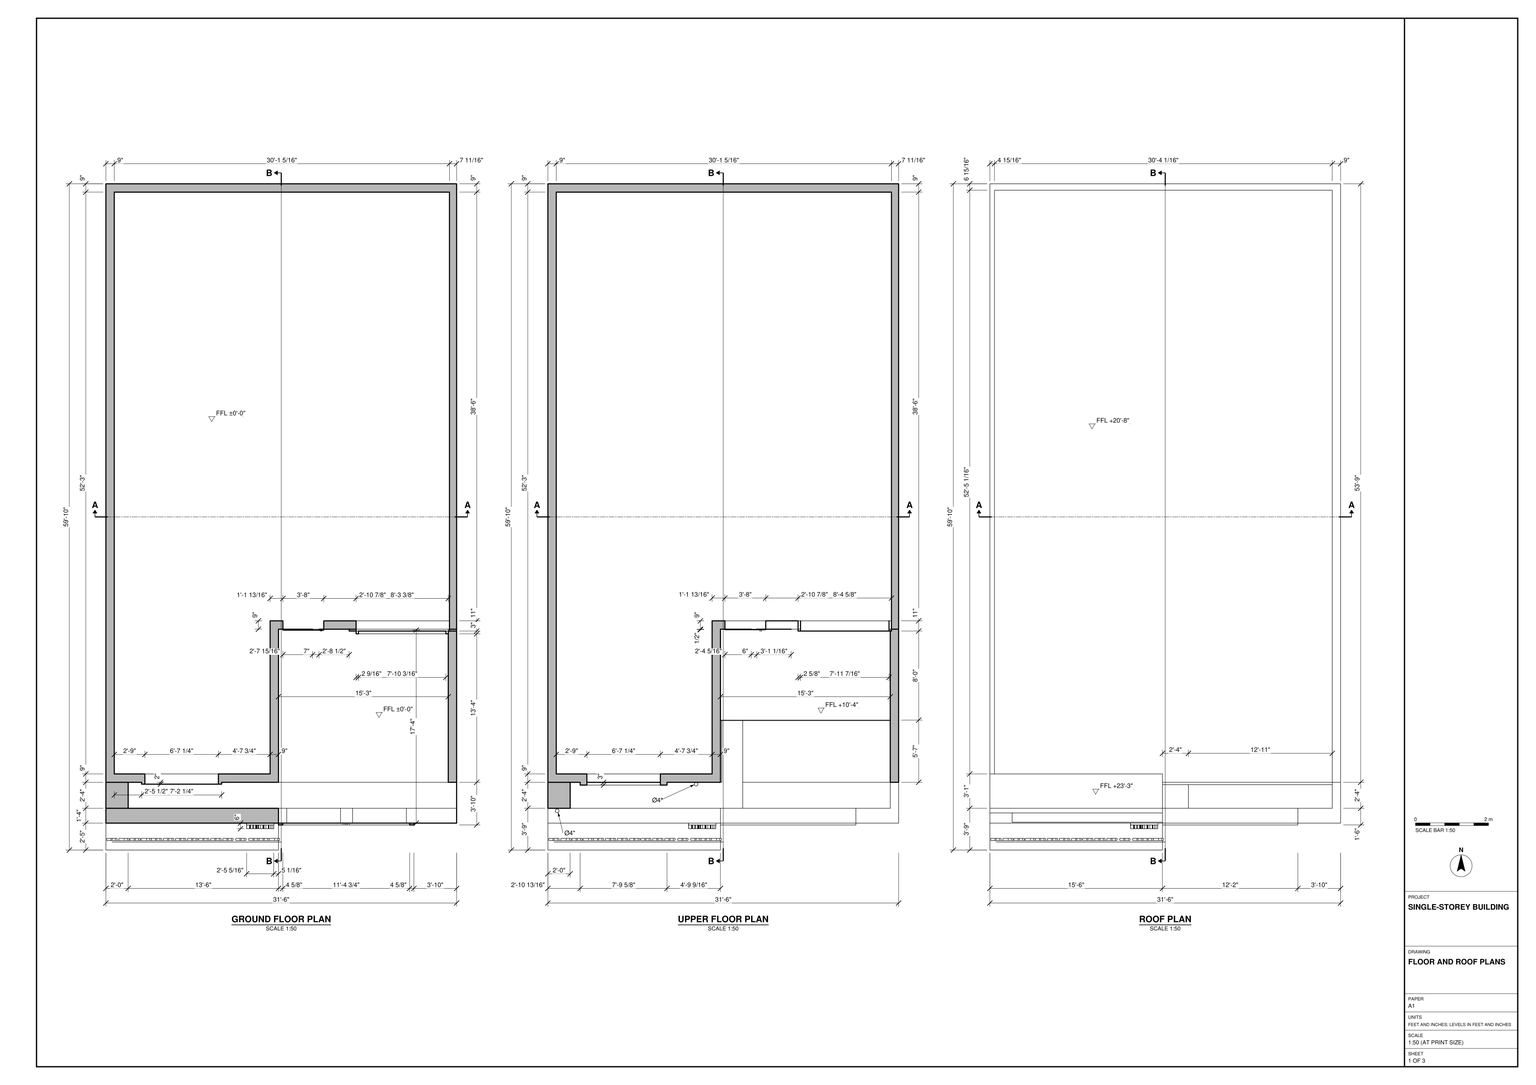
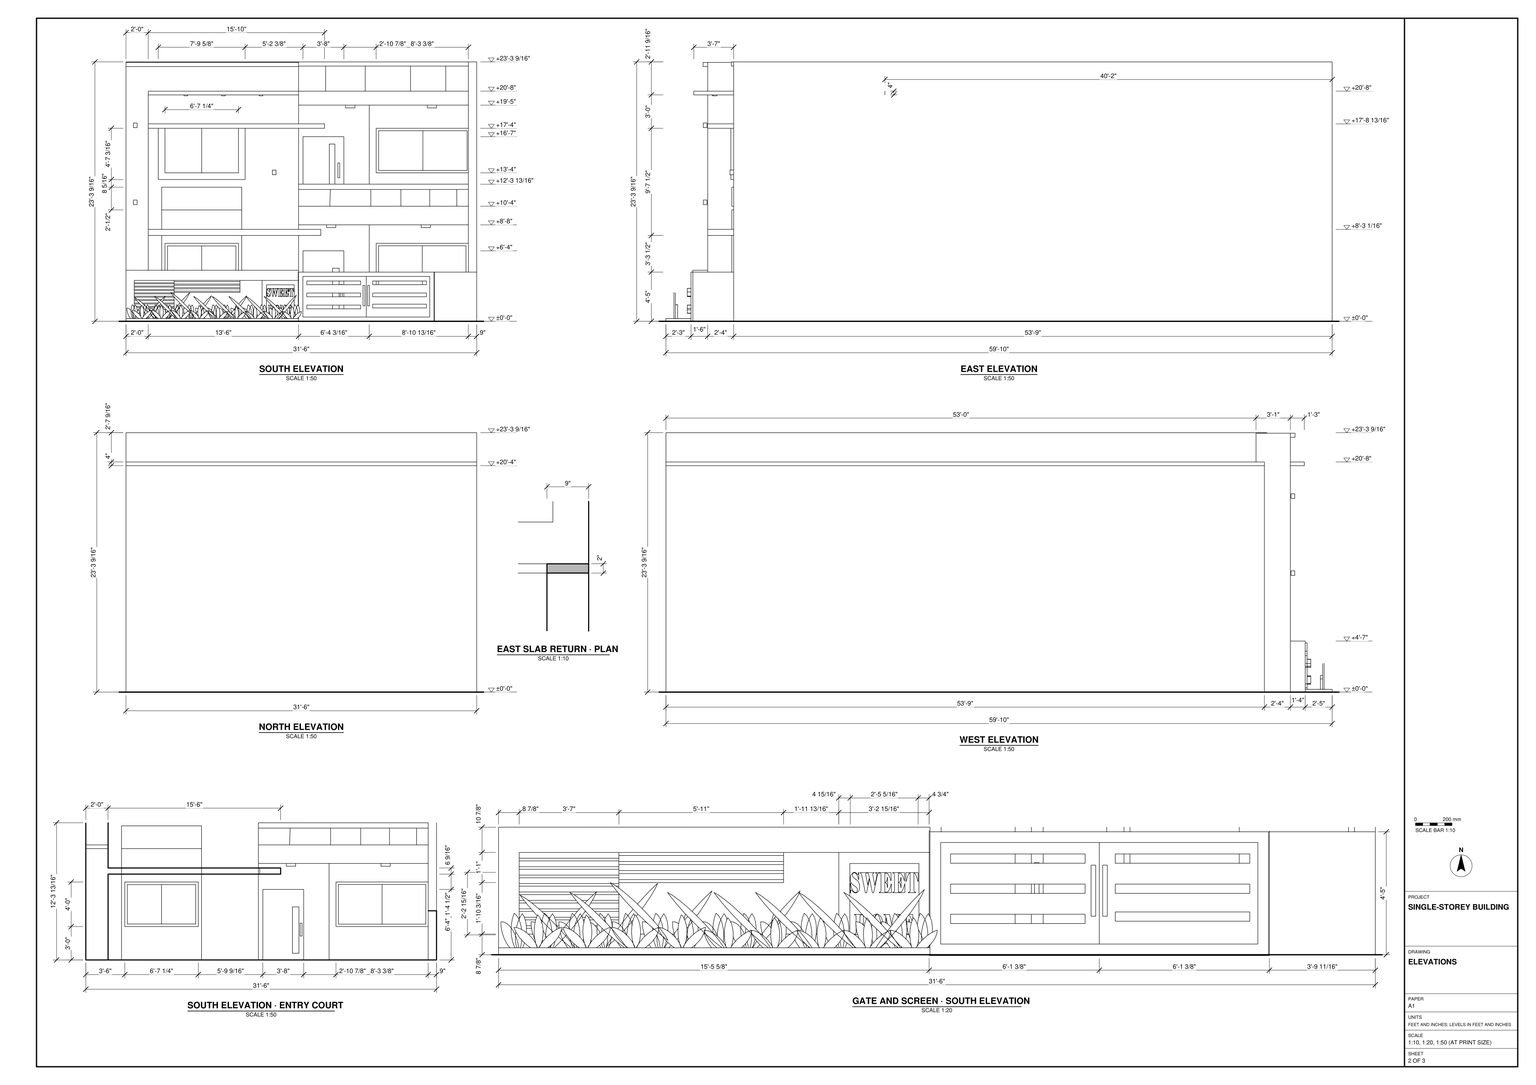
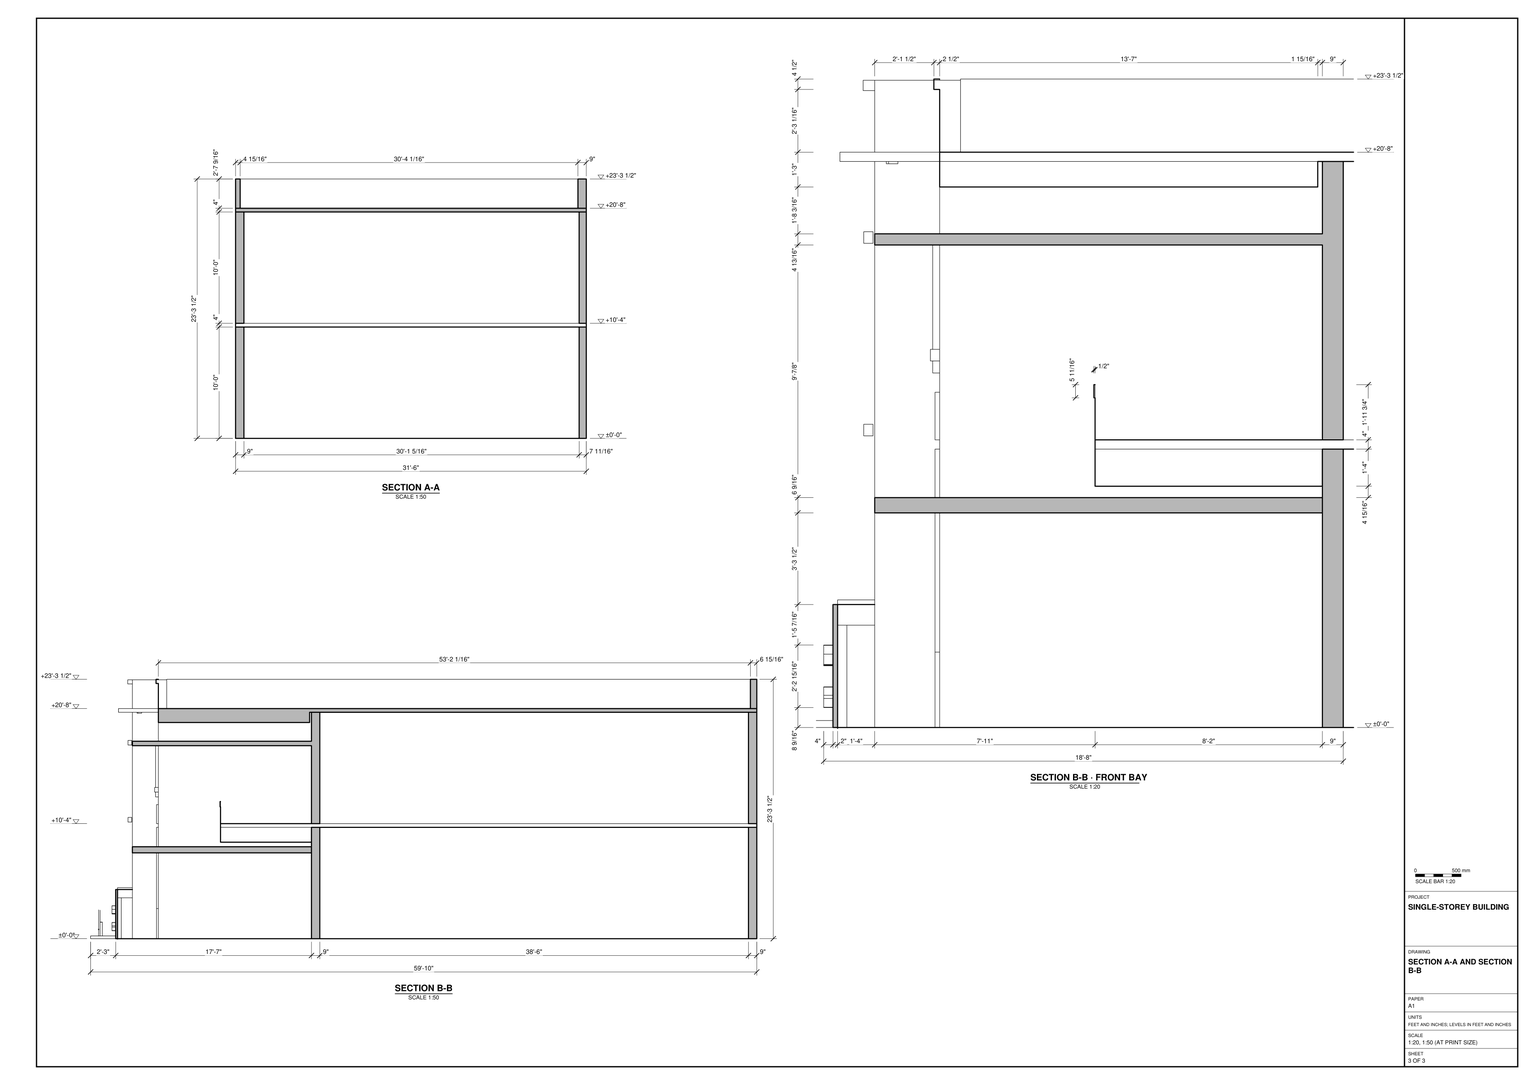
Build the house and its south entry court in SketchUp from task_files/diagram_01.pdf. Work in feet and inches. The overall model is 31'-6" across the frontage, 59'-10" from front to back and 23'-3 7/8" high. Set the ground floor at ±0'-0", the upper floor at +10'-4" and the main roof surface at +20'-8".

Use the floor plans to lay out the long side walls, the rear wall and the stepped south frontage. Follow the wall thicknesses as drawn. The west bay extends toward the street, while the door and wide window to its east sit farther back in the court. Use the sections to distinguish the upper floor slab and its projection into the court from the thinner shading ledges. Model the flat roof and its raised parapet. Use the south elevations to place the framed windows, doors and projecting bands at both storeys.

At the street edge, model the screen and its planting strip on the left and the paired gate leaves on the right, as seen from the south. Decor and loose items, including the plants, may be any suitable library components. Keep walls, slabs, roof elements and individual fitted pieces in separate groups or components, and use components for repeated parts. Save one SketchUp model as output_files/two_storey_house_with_a_screened_entry_court.skp.

# SketchUp Ruby script. Lengths in inches.
U = 1.inch
M = Sketchup.active_model
def pt(a) = Geom::Point3d.new(a.map { |v| v * U })
def face(e, loops, mat)
  f = e.add_face(loops[0].map { |a| pt(a) })
  loops[1..].each { |l| e.add_face(l.map { |a| pt(a) }).erase! }
  f.material = f.back_material = mat if mat
  f
end
# faces: each face lists its corners as indices into pts; further lists are holes
def faces(e, pts, list, mat = nil) = list.each { |f| face(e, (f[0].is_a?(Array) ? f : [f]).map { |l| l.map { |i| pts[i] } }, mat) }
# xy, xz, yz: faces in a plane at the given z, y or x. An outline is a flat list of corners, or four numbers for a rectangle; further outlines are holes
def ring(l) = l.size == 4 ? [[l[0], l[1]], [l[2], l[1]], [l[2], l[3]], [l[0], l[3]]] : l.each_slice(2).to_a
def flat(e, list, mat, &to3) = list.each { |f| face(e, (f[0].is_a?(Array) ? f : [f]).map { |l| ring(l).map { |u, v| to3.(u, v) } }, mat) }
def xy(e, z, list, mat = nil) = flat(e, list, mat) { |x, y| [x, y, z] }
def xz(e, y, list, mat = nil) = flat(e, list, mat) { |x, z| [x, y, z] }
def yz(e, x, list, mat = nil) = flat(e, list, mat) { |y, z| [x, y, z] }
def lines(e, pts, list) = list.each { |a, b| e.add_line(pt(pts[a]), pt(pts[b])) }
# prism: a flat outline (further loops are holes) pulled along v
def prism(e, loops, v, mat = nil)
  f = face(e, loops, mat); d = Geom::Vector3d.new(v.map { |x| x * U })
  f.pushpull(f.normal.samedirection?(d) ? d.length : -d.length)
end
def box(e, o, s, mat = nil) = prism(e, [[o, [o[0] + s[0], o[1], o[2]], [o[0] + s[0], o[1] + s[1], o[2]], [o[0], o[1] + s[1], o[2]]]], [0, 0, s[2]], mat)
def at(x, y, z, deg = 0) = Geom::Transformation.translation(pt([x, y, z])) * Geom::Transformation.rotation(ORIGIN, Z_AXIS, deg.degrees)
def axes(o, x, y, z) = Geom::Transformation.new([*x, 0, *y, 0, *z, 0, *pt(o).to_a, 1])
def part(name) = M.definitions.add(name)
# library, detail: a bought-in or finely detailed component or shape, given as its bounding box
def library(name, o, s) = part(name).tap { |d| box(d.entities, o, s) }
def detail(e, o, s) = box(e.add_group.entities, o, s)
def put(e, d, t, mat = nil) = e.add_instance(d, t).tap { |i| i.material = mat if mat }
def group(e, t, mat = nil) = e.add_group.tap { |g| g.transformation = t; g.material = mat if mat }.entities
root = M.entities
M.materials.add("Lily_Dark").color = [68, 42, 38]
M.materials.add("[Cladding Siding Tan]").color = [162, 126, 95]
M.materials.add("[Cladding Siding White]").color = [207, 207, 207]
M.materials.add("[Color A02]").color = [255, 153, 153]
M.materials.add("[Color C01]").color = [255, 229, 204]
M.materials.add("[Color D03]").color = [255, 216, 101]
M.materials.add("[Color M00]").color = [255, 255, 255]
M.materials.add("[Color M09]").color = [0, 0, 0]
M.materials.add("[Formica Speckled Grey]").color = [94, 105, 111]
M.materials.add("[Grass Dark Green]").color = [106, 157, 55]
M.materials.add("[Quartz Light Brown]").color = [199, 184, 152]
M.materials.add("[Translucent Glass Gray]").color = [128, 128, 128]
M.materials["[Translucent Glass Gray]"].alpha = 0.5
M.materials.add("[Vegetation Blur 03]").color = [83, 114, 18]
M.materials.add("[Vegetation Grass Artificial]").color = [98, 140, 74]
M.materials.add("[Vegetation Grass]").color = [144, 160, 91]
M.materials.add("[Wood Cherry Original]").color = [152, 86, 42]
M.materials.add("[Wood Lumber ButtJoined]").color = [164, 152, 112]
M.materials.add("[Wood Veneer 01]").color = [120, 70, 37]
M.materials.add("[Wood Veneer 02]").color = [190, 128, 91]
c1 = part("Horizontal screen slat")
box(c1.entities,[0,0,0],[42.97,1,2.5])
c2 = part("Slatted screen panel")
put(c2.entities,c1,at(0,-1,0),"[Wood Cherry Original]")
put(c2.entities,c1,at(0,-1,-3.63),"[Wood Cherry Original]")
put(c2.entities,c1,at(0,-1,-7.27),"[Wood Cherry Original]")
put(c2.entities,c1,at(0,-1,-10.9),"[Wood Cherry Original]")
put(c2.entities,c1,at(0,-1,-14.53),"[Wood Cherry Original]")
put(c2.entities,c1,at(0,-1,-18.17),"[Wood Cherry Original]")
put(c2.entities,c1,at(0,-1,-21.8),"[Wood Cherry Original]")
put(c2.entities,c1,at(0,-1,-25.43),"[Wood Cherry Original]")
put(c2.entities,c1,at(0,-1,-29.07),"[Wood Cherry Original]")
put(c2.entities,c1,at(0,-1,-32.7),"[Wood Cherry Original]")
c3 = library("SWEET  HOME",[-3.58,-8.11,0],[25.68,26.97,6])
c4 = part("Difference\#1")
xy(c4.entities,0,[[38.49,-2,38.49,0,0,0,0,645,378,645,378,165,234.81,165,234.81,174,370.29,174,370.29,636,9,636,9,9,177,9,177,174,190.8,174,190.8,165,186,165,186,0,124.73,0,124.73,-2]],"[Cladding Siding White]")
xy(c4.entities,20.51,[[38.49,-2,124.73,0]],"[Cladding Siding Tan]")
xy(c4.entities,28.81,[[34.8,-3,128.41,0]],"[Cladding Siding White]")
xy(c4.entities,36,[[42,-3,121.22,0],[42,0,121.22,9],[269.66,165,370.29,174]],"[Cladding Siding White]")
xy(c4.entities,75,[[190.8,165,234.81,174]],"[Cladding Siding White]")
xy(c4.entities,84,[[34.8,-3,42,0],[121.22,-3,128.41,0],[42,0,121.22,9],[269.66,165,370.29,174]],"[Cladding Siding White]")
xy(c4.entities,84,[[24,-28,24,0,34.8,0,34.8,-3,42,-3,42,0,121.22,0,121.22,-3,128.41,-3,128.41,0,186,0,186,165,214,165,214,-28]],"[Color M00]")
xy(c4.entities,88.8125,[[24,-28,214,-28,214,165,186,165,186,0,24,0]],"[Color M00]")
xy(c4.entities,120,[[[0,0,186,0,186,165,378,165,378,645,0,645],[9,9,9,636,370.29,636,370.29,174,177,174,177,9]]],"[Cladding Siding White]")
xz(c4.entities,-28,[[24,84,214,88.8125]],"[Color M00]")
xz(c4.entities,-3,[[34.8,28.81,128.41,28.81,128.41,84,121.22,84,121.22,36,42,36,42,84,34.8,84]],"[Formica Speckled Grey]")
xz(c4.entities,-2,[[38.49,0,124.73,20.51]],"[Cladding Siding Tan]")
xz(c4.entities,0,[[0,0,38.49,0,38.49,20.51,124.73,20.51,124.73,0,186,0,186,84,128.41,84,128.41,28.81,34.8,28.81,34.8,84,24,84,24,88.8125,186,88.8125,186,120,0,120]])
xz(c4.entities,0,[[24,84,34.8,88.8125],[34.8,84,128.41,88.8125]],"[Cladding Siding White]")
xz(c4.entities,9,[[[9,0,177,120],[42,36,121.22,84]]],"[Cladding Siding White]")
xz(c4.entities,165,[[190.8,84,214,88.8125],[190.8,84,214,88.8125]],"[Cladding Siding White]")
xz(c4.entities,165,[[186,0,190.8,0,190.8,75,234.81,75,234.81,0,262.2,0,262.2,120,186,120,186,88.8125,214,88.8125,214,84,186,84]],"[Color C01]")
xz(c4.entities,174,[[177,0,177,120,370.29,120,370.29,84,269.66,84,269.66,36,370.29,36,370.29,0,234.81,0,234.81,75,190.8,75,190.8,0]],"[Cladding Siding White]")
xz(c4.entities,636,[[9,0,370.29,120]],"[Cladding Siding White]")
xz(c4.entities,645,[[0,0,378,120]],"[Color C01]")
yz(c4.entities,0,[[0,0,645,120]],"[Color C01]")
yz(c4.entities,9,[[9,0,636,120]],"[Color C01]")
yz(c4.entities,24,[[-28,84,0,88.8125]],"[Cladding Siding White]")
yz(c4.entities,34.8,[[-3,28.81,0,84]],"[Cladding Siding White]")
yz(c4.entities,38.49,[[-2,0,0,20.51]],"[Cladding Siding Tan]")
yz(c4.entities,42,[[-3,36,0,84],[0,36,9,84]],"[Cladding Siding White]")
yz(c4.entities,121.22,[[-3,36,0,84],[0,36,9,84]],"[Cladding Siding White]")
yz(c4.entities,124.73,[[-2,0,0,20.51]],"[Cladding Siding Tan]")
yz(c4.entities,128.41,[[-3,28.81,0,84]],"[Cladding Siding White]")
yz(c4.entities,177,[[9,0,174,120]],"[Cladding Siding White]")
yz(c4.entities,186,[[0,0,165,84],[0,88.8125,165,120]],"[Color C01]")
yz(c4.entities,190.8,[[165,0,174,75]],"[Color C01]")
yz(c4.entities,214,[[-28,84,165,88.8125]],"[Color M00]")
yz(c4.entities,234.81,[[165,0,174,75]],"[Cladding Siding White]")
yz(c4.entities,269.66,[[165,36,174,84]],"[Cladding Siding White]")
yz(c4.entities,370.29,[[174,0,636,120],[165,36,174,84]],"[Cladding Siding White]")
yz(c4.entities,378,[[165,0,645,120]],"[Color C01]")
c5 = part("Horizontal screen slat \#1")
box(c5.entities,[0,0,0],[71,1,1.32])
c6 = part("Slatted screen panel \#1")
put(c6.entities,c5,at(0,-1,0))
put(c6.entities,c5,at(0,-1,-3.89))
put(c6.entities,c5,at(0,-1,-7.78))
put(c6.entities,c5,at(0,-1,-11.68))
c7 = part("Group\#6")
prism(c7.entities,[[[5.125,1,46.375],[9.35,1,43.61],[12.97,1,39.2],[15.75,1,33.46],[17.5,1,26.78],[18.1,1,19.6],[17.5,1,12.43],[15.75,1,5.74],[12.97,1,0],[8.75,1,2.77],[5.125,1,7.17],[2.34,1,12.92],[0.6,1,19.6],[0,1,26.78],[0.6,1,33.95],[2.34,1,40.64]]],[0,-1,0])
c8 = part("Group\#10")
put(c8.entities,c7,axes([18.75,0,-5.5],[0.86603,0,0.5],[0,1,0],[-0.5,0,0.86603]),"[Vegetation Blur 03]")
put(c8.entities,c7,at(17.01,0,0.98),"[Vegetation Blur 03]")
put(c8.entities,c7,axes([18.59,0,3.36],[0.96593,0,-0.25882],[0,1,0],[0.25882,0,0.96593]),"[Vegetation Blur 03]")
c9 = part("Group\#8")
xz(c9.entities,0,[[1.77,0,1.88,0.48,2.48,4.63,2.86,9.46,2.98,14.65,2.86,19.84,2.48,24.67,1.88,28.82,1.78,29.24,1.22,27.6,0.65,24.72,0.24,21.15,0.02,17.13,0,12.95,0.18,8.88,0.56,5.21,1.1,2.18]])
c10 = part("Group\#17")
put(c10.entities,c9,axes([1.625,0,12.02],[-0.91924,0,-0.91924],[0,1,0],[0.35492,0,-0.35492]),"[Vegetation Grass Artificial]")
put(c10.entities,c9,axes([12.49,0,15.8],[-1.29995,0,-0.01122],[0,1,0],[0.00433,0,-0.50192]),"[Vegetation Grass Artificial]")
put(c10.entities,c9,axes([22.13,0,8.8],[-0.91924,0,0.91924],[0,1,0],[-0.35492,0,-0.35492]),"[Vegetation Grass Artificial]")
c11 = part("Difference\#2")
xy(c11.entities,0,[[38.49,-2,38.49,0,0,0,0,645,378,645,378,165,234.81,165,234.81,174,370.29,174,370.29,636,9,636,9,9,177,9,177,174,190.8,174,190.8,165,186,165,186,0,124.73,0,124.73,-2]])
xy(c11.entities,0,[[262.18,163,378,165]],"[Cladding Siding White]")
xy(c11.entities,36,[[42,-2,121.22,9],[269.66,165,370.29,174]])
xy(c11.entities,36,[[269.66,163,370.29,165]],"[Cladding Siding White]")
xy(c11.entities,76,[[190.8,165,234.81,174]])
xy(c11.entities,84,[[42,-2,121.22,9],[269.66,165,370.29,174]])
xy(c11.entities,84,[[269.66,163,370.29,165]],"[Cladding Siding White]")
xy(c11.entities,120,[[38.49,-2,124.73,0],[[0,0,186,0,186,165,378,165,378,645,0,645],[9,9,9,636,370.29,636,370.29,174,177,174,177,9]]])
xy(c11.entities,120,[[262.18,163,378,165]],"[Cladding Siding White]")
xz(c11.entities,-2,[[[38.49,0,124.73,120],[42,36,121.22,84]]],"[Cladding Siding Tan]")
xz(c11.entities,0,[[0,0,38.49,120],[124.73,0,186,120],[38.49,120,124.73,144.51]])
xz(c11.entities,9,[[[9,0,177,120],[42,36,121.22,84]]])
xz(c11.entities,163,[[[262.18,0,378,120],[269.66,36,370.29,84]]],"[Cladding Siding Tan]")
xz(c11.entities,165,[[[262.18,0,378,120],[269.66,36,370.29,84]]],"[Cladding Siding White]")
xz(c11.entities,165,[[186,0,190.8,0,190.8,76,234.81,76,234.81,0,262.18,0,262.18,120,186,120]],"[Color C01]")
xz(c11.entities,174,[[177,0,177,120,370.29,120,370.29,84,269.66,84,269.66,36,370.29,36,370.29,0,234.81,0,234.81,76,190.8,76,190.8,0]])
xz(c11.entities,636,[[9,0,370.29,120]])
xz(c11.entities,645,[[0,0,378,120]],"[Color C01]")
yz(c11.entities,0,[[0,0,645,120]],"[Color C01]")
yz(c11.entities,9,[[9,0,636,120]])
yz(c11.entities,38.49,[[-2,0,0,32.49],[-2,32.49,0,120]])
yz(c11.entities,42,[[-2,36,9,84]])
yz(c11.entities,121.22,[[-2,36,9,84]])
yz(c11.entities,124.73,[[-2,0,0,32.49],[-2,32.49,0,120]])
yz(c11.entities,177,[[9,0,174,120]])
yz(c11.entities,186,[[0,0,165,120]],"[Color C01]")
yz(c11.entities,190.8,[[165,0,174,76]])
yz(c11.entities,234.81,[[165,0,174,76]])
yz(c11.entities,262.18,[[163,0,165,120]],"[Cladding Siding Tan]")
yz(c11.entities,269.66,[[165,36,174,84]])
yz(c11.entities,269.66,[[163,36,165,84]],"[Cladding Siding White]")
yz(c11.entities,370.29,[[174,0,636,120],[165,36,174,84]])
yz(c11.entities,370.29,[[163,36,165,84]],"[Cladding Siding White]")
yz(c11.entities,378,[[165,0,645,120]],"[Color C01]")
xy(root,0,[[146.68,29,186,33],[186,29,378,45],[0,45,24,73],[24,45,378,73],[0,73,369.01,73,369.01,238,378,238,378,718,0,718],
  [190.8,237,234.81,238]])
xy(root,0,[[186,27,331.97,29]],"Lily_Dark")
xy(root,0,[[0,29,0,45,186,45,186,33,146.68,33,146.68,29]],"[Formica Speckled Grey]")
xy(root,3,[[0,0,186,29]],"[Vegetation Grass]")
xy(root,4.61,[[190.61,27,258.99,29],[258.99,27,327.36,29]])
xy(root,4.76,[[151.4375,27,181.24,29],[151.4375,29,181.24,33]])
xy(root,7.2,[[222.71,237,229.71,238]])
xy(root,8.9,[[8.9,29,146.68,33]],"[Formica Speckled Grey]")
xy(root,13.46,[[194.88,29,252.88,45]])
xy(root,14.46,[[265.88,29,323.88,45]])
xy(root,16.625,[[255.45,27,257.45,29],[260.45,27,262.45,29]],"[Color M09]")
xy(root,17.46,[[194.88,29,252.88,45]])
xy(root,18.46,[[265.88,29,323.88,45]])
xy(root,25.72,[[231.03,237,233.03,238]])
xy(root,26.46,[[194.88,29,252.88,45],[265.88,29,323.88,45]])
xy(root,30.46,[[194.88,29,252.88,45],[265.88,29,323.88,45]])
xy(root,33.72,[[231.03,237,233.03,238]])
xy(root,36,[[42,71,121.22,82],[269.66,233,269.66,247,370.29,247,370.29,238,369.01,238,369.01,233],[369.01,236,370.29,238]])
xy(root,38.57,[[272.23,233,366.44,236]])
xy(root,38.625,[[255.45,27,257.45,29],[260.45,27,262.45,29]],"[Color M09]")
xy(root,39.34,[[151.4375,27,181.24,29],[151.4375,29,181.24,33]])
xy(root,39.46,[[194.88,29,252.88,45]])
xy(root,39.72,[[231.03,236,233.03,237]],"[Color M09]")
xy(root,43.46,[[194.88,29,252.88,45]])
xy(root,44.1,[[146.68,29,186,33]])
xy(root,44.1,[[8.9,29,146.68,33]],"[Formica Speckled Grey]")
xy(root,48.39,[[190.61,27,258.99,29],[258.99,27,327.36,29]])
xy(root,53,[[186,27,331.97,29],[186,29,331.97,45]],"Lily_Dark")
xy(root,53,[[331.97,29,378,29,378,73,369.01,73,369.01,45,331.97,45]],"[Color C01]")
xy(root,55,[[0,29,186,45]],"[Formica Speckled Grey]")
xy(root,57.2,[[222.71,237,229.71,238]])
xy(root,76,[[190.8,237,234.81,238]])
xy(root,81.43,[[272.23,233,366.44,236]])
xy(root,84,[[42,71,121.22,82],[269.66,233,369.01,233,369.01,238,370.29,238,370.29,247,269.66,247],[369.01,236,370.29,238]])
xy(root,92.52,[[24,45,24,73,187.45,73,187.45,238,210,238,210,45]])
xy(root,99.09,[[24,45,210,45,210,238,187.45,238,187.45,73,24,73]])
xy(root,124,[[190.8,237.5,234.81,238]])
xy(root,128.07,[[219.14,237.5,225.14,238]])
xy(root,154.6875,[[228.35,236,230.35,237.5],[228.35,237.5,230.35,238]])
xy(root,160,[[269.66,236,269.66,247,370.29,247,370.29,238,369.01,238,369.01,236],[369.01,236,370.29,238]])
xy(root,162.61,[[272.26,236,367.68,247]])
xy(root,170.6875,[[228.35,236,230.35,237.5],[228.35,237.5,230.35,238]])
xy(root,191.07,[[219.14,237.5,225.14,238]])
xy(root,199,[[190.8,237.5,234.81,238]])
xy(root,205.39,[[272.26,236,367.68,247]])
xy(root,208,[[269.66,236,369.01,236,369.01,238,370.29,238,370.29,247,269.66,247],[369.01,236,370.29,238]])
xy(root,243,[[64.5,50,63.98,50.07,63.5,50.27,63.09,50.59,62.77,51,62.57,51.48,62.5,52,62.57,52.52,62.77,53,63.09,53.41,63.5,53.73,63.98,53.93,64.5,54,65.02,53.93,65.5,53.73,65.91,53.41,66.23,53,66.43,52.52,66.5,52,66.43,51.48,66.23,51,65.91,50.59,65.5,50.27,65.02,50.07],[105,51,104.48,51.07,104,51.27,103.59,51.59,103.27,52,103.07,52.48,103,53,103.07,53.52,103.27,54,103.59,54.41,104,54.73,104.48,54.93,105,55,105.52,54.93,106,54.73,106.41,54.41,106.73,54,106.93,53.52,107,53,106.93,52.48,106.73,52,106.41,51.59,106,51.27,105.52,51.07],[145.5,51,144.98,51.07,144.5,51.27,144.09,51.59,143.77,52,143.57,52.48,143.5,53,143.57,53.52,143.77,54,144.09,54.41,144.5,54.73,144.98,54.93,145.5,55,146.02,54.93,146.5,54.73,146.91,54.41,147.23,54,147.43,53.52,147.5,53,147.43,52.48,147.23,52,146.91,51.59,146.5,51.27,146.02,51.07]],"[Color D03]")
xy(root,244,[[[24,30,186,73],[145.5,51,146.02,51.07,146.5,51.27,146.91,51.59,147.23,52,147.43,52.48,147.5,53,147.43,53.52,147.23,54,146.91,54.41,146.5,54.73,146.02,54.93,145.5,55,144.98,54.93,144.5,54.73,144.09,54.41,143.77,54,143.57,53.52,143.5,53,143.57,52.48,143.77,52,144.09,51.59,144.5,51.27,144.98,51.07],[105,51,105.52,51.07,106,51.27,106.41,51.59,106.73,52,106.93,52.48,107,53,106.93,53.52,106.73,54,106.41,54.41,106,54.73,105.52,54.93,105,55,104.48,54.93,104,54.73,103.59,54.41,103.27,54,103.07,53.52,103,53,103.07,52.48,103.27,52,103.59,51.59,104,51.27,104.48,51.07],[64.5,50,65.02,50.07,65.5,50.27,65.91,50.59,66.23,51,66.43,51.48,66.5,52,66.43,52.52,66.23,53,65.91,53.41,65.5,53.73,65.02,53.93,64.5,54,63.98,53.93,63.5,53.73,63.09,53.41,62.77,53,62.57,52.52,62.5,52,62.57,51.48,62.77,51,63.09,50.59,63.5,50.27,63.98,50.07]]])
xy(root,248,[[24,30,186,45],[24,45,186,73],[0,82,0,718,378,718,378,238,369.01,238,369.01,711.09,4.95,711.09,4.95,82]])
xy(root,275.04,[[186,70.5,369.01,73]])
xy(root,279,[[0,45,186,82]])
xy(root,279.54,[[369.01,73,378,73,378,718,0,718,0,82,4.95,82,4.95,711.09,369.01,711.09]])
xy(root,279.54,[[186,70.5,369.01,73]],"[Formica Speckled Grey]")
xz(root,0,[[0,0,186,3]],"[Vegetation Grass]")
xz(root,27,[[151.4375,4.76,181.24,39.34]])
xz(root,27,[[[186,0,331.97,53],[190.61,4.61,327.36,48.39]]],"Lily_Dark")
xz(root,27,[[255.45,16.625,257.45,38.625],[260.45,16.625,262.45,38.625]],"[Color M09]")
xz(root,29,[[185.64,-0.36,332.33,0],[[186,0,331.97,53],[190.61,4.61,327.36,48.39]]])
xz(root,29,[[331.97,0,332.33,53],[332.33,0,378,53]],"[Color C01]")
xz(root,29,[[0,3,146.68,3,146.68,8.9,8.9,8.9,8.9,44.1,185.64,44.1,185.64,53.36,186,53.36,186,55,0,55],[[146.68,3,185.64,44.1],[151.4375,4.76,181.24,39.34]],[185.64,3,186,44.1],[185.64,44.1,186,53.36]],"[Formica Speckled Grey]")
xz(root,29,[[[190.61,4.61,258.99,48.39],[194.88,39.46,252.88,43.46],[194.88,26.46,252.88,30.46],[194.88,13.46,252.88,17.46],[255.45,16.625,257.45,38.625]],[[258.99,4.61,327.36,48.39],[265.88,39.46,323.88,43.46],[265.88,26.46,323.88,30.46],[265.88,14.46,323.88,18.46],[260.45,16.625,262.45,38.625]]],"[Quartz Light Brown]")
xz(root,29,[[0,0,146.68,3],[146.68,0,185.64,3],[185.64,0,186,3]],"[Vegetation Grass]")
xz(root,30,[[24,244,186,248]])
xz(root,33,[[[146.68,0,186,44.1],[151.4375,4.76,181.24,39.34]],[8.9,8.9,51.87,41.6],[8.9,41.6,51.87,44.1]])
xz(root,33,[[51.87,8.9,146.68,8.9,146.68,44.1,122.87,44.1,122.87,31.1,51.87,31.1]],"[Color C01]")
xz(root,45,[[0,0,24,55],[24,0,186,55],[24,92.52,210,99.09]])
xz(root,45,[[0,55,24,55,24,248,186,248,186,274.56,0,274.56]],"[Formica Speckled Grey]")
xz(root,70.5,[[186,275.04,369.01,279.54]],"[Formica Speckled Grey]")
xz(root,71,[[[42,36,121.22,84],[44.76,38.77,118.46,81.23]]],"[Formica Speckled Grey]")
xz(root,71,[[44.76,38.77,81.61,81.23],[81.61,38.77,118.46,81.23]],"[Translucent Glass Gray]")
xz(root,73,[[369.01,0,378,53],[24,208,42,212.8125],[42,208,186,212.8125],[24,244,186,248]])
xz(root,73,[[369.01,53,378,279.54]],"[Color C01]")
xz(root,73,[[42,160,81.61,208],[81.61,160,121.22,208],[186,248,215.2,275.04],[215.2,248,257.85,275.04],[257.85,248,306.66,275.04],
  [306.66,248,344.64,275.04],[344.64,248,369.01,275.04]],"[Translucent Glass Gray]")
xz(root,82,[[4.95,248,186,279]])
xz(root,82,[[0,248,4.95,279],[0,279,4.95,279.54]],"[Color C01]")
xz(root,233,[[[269.66,36,369.01,84],[272.23,38.57,366.44,81.43]]],"[Formica Speckled Grey]")
xz(root,236,[[369.01,36,370.29,84]])
xz(root,236,[[231.03,25.72,233.03,39.72],[228.35,154.6875,230.35,170.6875]],"[Color M09]")
xz(root,236,[[[269.66,160,369.01,208],[272.26,162.61,367.68,205.39]],[369.01,160,370.29,208]],"[Formica Speckled Grey]")
xz(root,236,[[272.23,38.57,319.33,81.43],[319.33,38.57,366.44,81.43],[272.26,162.61,319.97,205.39],[319.97,162.61,367.68,205.39]],"[Translucent Glass Gray]")
xz(root,237,[[231.03,33.72,233.03,39.72]],"[Color M09]")
xz(root,237,[[222.71,7.2,229.71,57.2]],"[Wood Lumber ButtJoined]")
xz(root,237,[[[190.8,0,234.81,76],[222.71,7.2,229.71,57.2],[231.03,25.72,233.03,39.72]]],"[Wood Veneer 01]")
xz(root,237.5,[[219.14,128.07,225.14,191.07]],"[Wood Lumber ButtJoined]")
xz(root,237.5,[[[190.8,124,234.81,199],[219.14,128.07,225.14,191.07],[228.35,154.6875,230.35,170.6875]]],"[Wood Veneer 01]")
xz(root,238,[[[190.8,0,234.81,76],[222.71,7.2,229.71,57.2],[231.03,25.72,233.03,33.72]],[369.01,0,369.01,36,370.29,36,370.29,84,369.01,84,369.01,120,378,120,378,0],[187.45,92.52,210,99.09],[369.01,120,378,124],[[190.8,124,234.81,199],[219.14,128.07,225.14,191.07],[228.35,154.6875,230.35,170.6875]],
  [369.01,124,369.01,160,370.29,160,370.29,208,369.01,208,369.01,248,378,248,378,124]])
xz(root,711.09,[[4.95,248,369.01,279.54]],"[Color C01]")
xz(root,718,[[0,248,378,279.54]])
yz(root,0,[[29,0,45,55],[45,0,45,279,82,279,82,248,73,248,73,0]])
yz(root,0,[[82,248,718,279.54]],"[Color C01]")
yz(root,0,[[0,0,29,3]],"[Vegetation Grass]")
yz(root,4.95,[[82,248,711.09,279.54]],"[Color C01]")
yz(root,8.9,[[29,8.9,33,44.1]],"[Formica Speckled Grey]")
yz(root,24,[[30,244,45,248]])
yz(root,24,[[45,0,73,92.52],[45,99.09,73,244]],"[Formica Speckled Grey]")
yz(root,42,[[71,36,82,84]])
yz(root,121.22,[[71,36,82,84]])
yz(root,146.68,[[29,0,33,8.9],[29,8.9,33,44.1]])
yz(root,151.4375,[[27,4.76,29,8.9],[29,4.76,33,8.9],[27,8.9,29,39.34],[29,8.9,33,39.34]])
yz(root,181.24,[[27,4.76,29,39.34],[29,4.76,33,39.34]])
yz(root,186,[[29,0,33,44.1],[33,0,45,44.1],[27,3,29,44.1],[27,44.1,29,53],[29,44.1,45,53],
  [73,208,238,212.8125],[30,244,73,248],[70.5,279,73,279.54]])
yz(root,186,[[29,53,45,55],[45,248,73,248,73,275.04,70.5,275.04,70.5,279,45,279],[73,248,82,248,82,279,70.5,279,70.5,275.04,73,275.04]],"[Formica Speckled Grey]")
yz(root,186,[[0,0,27,3],[27,0,29,3]],"[Vegetation Grass]")
yz(root,187.45,[[73,92.52,238,99.09]])
yz(root,190.61,[[27,4.61,29,44.1],[27,44.1,29,48.39]])
yz(root,190.8,[[237,0,238,76],[237.5,124,238,199]])
yz(root,194.88,[[29,13.46,45,17.46],[29,26.46,45,30.46],[29,39.46,45,43.46]])
yz(root,210,[[45,92.52,238,99.09]])
yz(root,219.14,[[237.5,128.07,238,191.07]])
yz(root,222.71,[[237,7.2,238,57.2]])
yz(root,225.14,[[237.5,128.07,238,191.07]])
yz(root,228.35,[[236,154.6875,237.5,170.6875],[237.5,154.6875,238,170.6875]])
yz(root,229.71,[[237,7.2,238,57.2]])
yz(root,230.35,[[236,154.6875,237.5,170.6875],[237.5,154.6875,238,170.6875]])
yz(root,231.03,[[236,25.72,237,39.72],[237,25.72,238,33.72]])
yz(root,233.03,[[236,25.72,237,39.72],[237,25.72,238,33.72]])
yz(root,234.81,[[237,0,238,76],[237.5,124,238,199]])
yz(root,252.88,[[29,13.46,45,17.46],[29,26.46,45,30.46],[29,39.46,45,43.46]])
yz(root,255.45,[[27,16.625,29,38.625]],"[Color M09]")
yz(root,257.45,[[27,16.625,29,38.625]],"[Color M09]")
yz(root,260.45,[[27,16.625,29,38.625]],"[Color M09]")
yz(root,262.45,[[27,16.625,29,38.625]],"[Color M09]")
yz(root,265.88,[[29,14.46,45,18.46],[29,26.46,45,30.46]])
yz(root,269.66,[[233,36,247,84],[236,160,247,208]])
yz(root,272.23,[[233,38.57,236,81.43]])
yz(root,272.26,[[236,162.61,247,205.39]])
yz(root,323.88,[[29,14.46,45,18.46],[29,26.46,45,30.46]])
yz(root,327.36,[[27,4.61,29,48.39]])
yz(root,331.97,[[27,0,29,53]])
yz(root,366.44,[[233,38.57,236,81.43]])
yz(root,367.68,[[236,162.61,247,205.39]])
yz(root,369.01,[[233,36,236,84],[70.5,275.04,73,279.54]])
yz(root,369.01,[[73,0,73,279.54,711.09,279.54,711.09,248,238,248,238,208,236,208,236,160,238,160,238,84,233,84,233,36,238,36,238,0]],"[Color C01]")
yz(root,370.29,[[236,36,238,84],[238,36,247,84],[236,160,238,208],[238,160,247,208]])
yz(root,378,[[29,0,73,53],[73,0,238,0,238,248,718,248,718,279.54,73,279.54]],"[Color C01]")
p = [[64.5,50,244],[63.98,50.07,244],[63.98,50.07,243],[64.5,50,243],[65.02,50.07,244],[65.02,50.07,243],
  [63.5,50.27,244],[63.5,50.27,243],[65.5,50.27,244],[65.5,50.27,243],[63.09,50.59,244],[63.09,50.59,243],
  [65.91,50.59,244],[65.91,50.59,243],[62.77,51,244],[62.77,51,243],[66.23,51,244],[66.23,51,243],
  [62.57,51.48,244],[62.57,51.48,243],[66.43,51.48,244],[66.43,51.48,243],[105,51,244],[104.48,51.07,244],
  [104.48,51.07,243],[105,51,243],[105.52,51.07,244],[105.52,51.07,243],[145.5,51,244],[144.98,51.07,244],
  [144.98,51.07,243],[145.5,51,243],[146.02,51.07,244],[146.02,51.07,243],[104,51.27,244],[104,51.27,243],
  [106,51.27,244],[106,51.27,243],[144.5,51.27,244],[144.5,51.27,243],[146.5,51.27,244],[146.5,51.27,243],
  [103.59,51.59,244],[103.59,51.59,243],[106.41,51.59,244],[106.41,51.59,243],[144.09,51.59,244],[144.09,51.59,243],
  [146.91,51.59,244],[146.91,51.59,243],[62.5,52,244],[62.5,52,243],[66.5,52,244],[66.5,52,243],
  [103.27,52,244],[103.27,52,243],[106.73,52,244],[106.73,52,243],[143.77,52,244],[143.77,52,243],
  [147.23,52,244],[147.23,52,243],[62.57,52.52,244],[62.57,52.52,243],[66.43,52.52,244],[66.43,52.52,243],
  [103.07,52.48,244],[103.07,52.48,243],[106.93,52.48,244],[106.93,52.48,243],[143.57,52.48,244],[143.57,52.48,243],
  [147.43,52.48,244],[147.43,52.48,243],[62.77,53,244],[62.77,53,243],[66.23,53,244],[66.23,53,243],
  [103,53,244],[103,53,243],[107,53,244],[107,53,243],[143.5,53,244],[143.5,53,243],
  [147.5,53,244],[147.5,53,243],[63.09,53.41,244],[63.09,53.41,243],[65.91,53.41,244],[65.91,53.41,243],
  [103.07,53.52,244],[103.07,53.52,243],[106.93,53.52,244],[106.93,53.52,243],[143.57,53.52,244],[143.57,53.52,243],
  [147.43,53.52,244],[147.43,53.52,243],[63.5,53.73,244],[63.5,53.73,243],[65.5,53.73,244],[65.5,53.73,243],
  [103.27,54,244],[103.27,54,243],[106.73,54,244],[106.73,54,243],[143.77,54,244],[143.77,54,243],
  [147.23,54,244],[147.23,54,243],[63.98,53.93,244],[63.98,53.93,243],[65.02,53.93,244],[65.02,53.93,243],
  [64.5,54,244],[64.5,54,243],[103.59,54.41,244],[103.59,54.41,243],[106.41,54.41,244],[106.41,54.41,243],
  [144.09,54.41,244],[144.09,54.41,243],[146.91,54.41,244],[146.91,54.41,243],[104,54.73,244],[104,54.73,243],
  [106,54.73,244],[106,54.73,243],[144.5,54.73,244],[144.5,54.73,243],[146.5,54.73,244],[146.5,54.73,243],
  [104.48,54.93,244],[104.48,54.93,243],[105.52,54.93,244],[105.52,54.93,243],[144.98,54.93,244],[144.98,54.93,243],
  [146.02,54.93,244],[146.02,54.93,243],[105,55,244],[105,55,243],[145.5,55,244],[145.5,55,243],
  [186,238,124],[190.8,238,124],[262.2,238,124],[369.01,238,124],[262.2,238,244],[234.81,238,124],
  [332.33,29,53],[332.33,29,53.36],[323.88,29,39.46],[323.88,45,39.46],[265.88,29,39.46],[265.88,45,39.46],
  [323.88,29,43.46],[323.88,45,43.46],[265.88,29,43.46],[265.88,45,43.46],[369.01,238,120],[186,238,120]]
faces(root,p,[[0,1,2,3],[4,0,3,5],[1,6,7,2],[8,4,5,9],[6,10,11,7],[12,8,9,13],[10,14,15,11],[16,12,13,17],
  [14,18,19,15],[20,16,17,21],[22,23,24,25],[26,22,25,27],[28,29,30,31],[32,28,31,33],[23,34,35,24],[36,26,27,37],
  [29,38,39,30],[40,32,33,41],[34,42,43,35],[44,36,37,45],[38,46,47,39],[48,40,41,49],[18,50,51,19],[52,20,21,53],
  [42,54,55,43],[56,44,45,57],[46,58,59,47],[60,48,49,61],[50,62,63,51],[64,52,53,65],[54,66,67,55],[68,56,57,69],
  [58,70,71,59],[72,60,61,73],[62,74,75,63],[76,64,65,77],[66,78,79,67],[80,68,69,81],[70,82,83,71],[84,72,73,85],
  [74,86,87,75],[88,76,77,89],[78,90,91,79],[92,80,81,93],[82,94,95,83],[96,84,85,97],[86,98,99,87],[100,88,89,101],
  [90,102,103,91],[104,92,93,105],[94,106,107,95],[108,96,97,109],[98,110,111,99],[112,100,101,113],[110,114,115,111],[114,112,113,115],
  [102,116,117,103],[118,104,105,119],[106,120,121,107],[122,108,109,123],[116,124,125,117],[126,118,119,127],[120,128,129,121],[130,122,123,131],
  [124,132,133,125],[134,126,127,135],[128,136,137,129],[138,130,131,139],[132,140,141,133],[140,134,135,141],[136,142,143,137],[142,138,139,143]],"[Color D03]")
lines(root,p,[[144,145],[146,147],[146,148],[149,146],[150,151],[152,153],[154,155],[156,157],[158,159],[160,161]])
detail(root,[236.75,147.12,230],[10,10,3])
detail(root,[324.73,147.12,230],[10,10,3])
detail(root,[216.12,176.17,101],[10,10,3])
detail(root,[318.12,176.17,101],[10,10,3])
detail(root,[8,40.27,125.71],[4,4,5])
detail(root,[8,40.27,208.71],[4,4,5])
detail(root,[157.72,69,158.01],[4,4,5])
put(root,c2,at(8.9,33,41.6))
put(root,c3,axes([155.71,29,16.69],[1.14,0,0],[0,0,1],[0,-1,0]),"[Color A02]")
g1 = group(root,at(0,73,120))
xy(g1,-16,[[186,67,186,165,378,163,378,67]],"[Formica Speckled Grey]")
xy(g1,0,[[38.49,-2,38.49,0,0,0,0,645,378,645,378,163,186,165,186,0,124.73,0,124.73,-2]])
xy(g1,4,[[186,67,378,165]],"[Formica Speckled Grey]")
xy(g1,22.11,[[186,66.5,378,67]])
xy(g1,27.8125,[[186,66.5,378,67]],"[Formica Speckled Grey]")
xz(g1,-2,[[38.49,0,124.73,4]],"[Cladding Siding Tan]")
xz(g1,0,[[0,0,24,4],[24,0,38.49,4],[124.73,0,186,4]])
xz(g1,66.5,[[186,22.11,378,27.8125]],"[Formica Speckled Grey]")
xz(g1,67,[[186,-16,378,4]],"[Formica Speckled Grey]")
xz(g1,67,[[186,4,219.62,4,220.25,22.11,186,22.11],[219.62,4,263.86,4,263.86,22.11,220.25,22.11],[263.86,4,296.28,22.11],[296.28,4,327.34,22.11],[327.34,4,356.51,22.11],
  [356.51,4,378,22.11]],"[Translucent Glass Gray]")
xz(g1,645,[[0,0,378,4]])
yz(g1,0,[[0,0,645,4]])
yz(g1,38.49,[[-2,0,0,4]],"[Cladding Siding Tan]")
yz(g1,124.73,[[-2,0,0,4]],"[Cladding Siding Tan]")
yz(g1,186,[[67,-16,165,0],[0,0,67,4],[66.5,22.11,67,27.8125]])
yz(g1,378,[[66.5,22.11,67,27.8125]])
yz(g1,378,[[67,-16,163,-16,163,0,645,0,645,4,67,4]],"[Color C01]")
p = [[186,165,0],[378,163,0],[378,163,-16],[186,165,-16]]
faces(g1,p,[[0,1,2,3]])
g2 = group(root,at(0,73,244))
xy(g2,-11,[[186,0,369.01,163]],"[Formica Speckled Grey]")
xy(g2,0,[[0,0,0,645,378,645,378,163,186,163,186,0]])
xy(g2,4,[[0,0,369.01,0,369.01,163,378,163,378,645,0,645]])
xz(g2,0,[[0,0,186,4]])
xz(g2,0,[[186,-11,369.01,4]],"[Formica Speckled Grey]")
xz(g2,163,[[186,-11,369.01,0],[369.01,0,378,4]])
xz(g2,645,[[0,0,378,4]])
yz(g2,0,[[0,0,645,4]])
yz(g2,186,[[0,-11,163,0]])
yz(g2,369.01,[[0,-11,163,4]])
yz(g2,378,[[163,0,645,4]])
put(root,c4,at(0,73,124),"[Color C01]")
g3 = group(root,at(0,45,274.56))
box(g3,[0,-5,0],[186,5,4.44])
g4 = group(root,at(8.9,33,8.9))
xz(g4,0,[[0,0,42.97,35.2]])
g5 = group(root,at(51.87,33,31.1))
xz(g5,0,[[0,0,71,11.68]])
put(g5,c6,at(0,0,11.68),"[Wood Veneer 02]")
put(root,c8,axes([0.99,12.6,0.7],[0.26,0,0],[0,-2.3983,0],[0,0,0.3633]))
put(root,c8,axes([13.99,12.6,0.7],[0.26,0,0],[0,-2.3983,0],[0,0,0.3633]))
put(root,c8,axes([25.99,12.6,0.7],[0.26,0,0],[0,-2.3983,0],[0,0,0.3633]))
put(root,c8,axes([37.99,12.6,0.7],[0.26,0,0],[0,-2.3983,0],[0,0,0.3633]))
put(root,c8,axes([48.99,12.6,0.7],[0.26,0,0],[0,-2.3983,0],[0,0,0.3633]))
put(root,c8,axes([61.99,12.6,0.7],[0.26,0,0],[0,-2.3983,0],[0,0,0.3633]))
put(root,c8,axes([74.99,12.6,0.7],[0.26,0,0],[0,-2.3983,0],[0,0,0.3633]))
put(root,c8,axes([87.99,12.6,0.7],[0.26,0,0],[0,-2.3983,0],[0,0,0.3633]))
put(root,c8,axes([99.99,12.6,0.7],[0.26,0,0],[0,-2.3983,0],[0,0,0.3633]))
put(root,c8,axes([112.99,12.6,0.7],[0.26,0,0],[0,-2.3983,0],[0,0,0.3633]))
put(root,c8,axes([125.99,12.6,0.7],[0.26,0,0],[0,-2.3983,0],[0,0,0.3633]))
put(root,c8,axes([139.99,12.6,0.7],[0.26,0,0],[0,-2.3983,0],[0,0,0.3633]))
put(root,c8,axes([153.99,12.6,0.7],[0.26,0,0],[0,-2.3983,0],[0,0,0.3633]))
put(root,c8,axes([164.99,12.6,0.7],[0.26,0,0],[0,-2.3983,0],[0,0,0.3633]))
g6 = group(root,at(175.99,12.6,0.7))
put(g6,c7,axes([4.875,0,-2],[0.22517,0,0.18165],[0,-2.3983,0],[-0.13,0,0.31463]),"[Vegetation Blur 03]")
put(g6,c7,axes([4.42,0,0.36],[0.26,0,0],[0,-2.3983,0],[0,0,0.3633]),"[Vegetation Blur 03]")
put(g6,c7,axes([4.83,0,1.22],[0.25114,0,-0.09403],[0,-2.3983,0],[0.06729,0,0.35092]),"[Vegetation Blur 03]")
put(root,c9,axes([10.53,10.2,26.97],[-0.70711,0,-0.70711],[0,1,0],[0.85107,0,-0.85107]),"[Grass Dark Green]")
put(root,c10,at(6.66,8.63,1.42))
put(root,c10,at(27.66,8.63,1.42))
put(root,c10,at(48.66,8.63,1.42))
put(root,c10,at(68.66,8.63,1.42))
put(root,c10,at(88.625,8.63,0.19))
put(root,c10,at(108.625,8.63,0.19))
put(root,c10,at(128.625,8.63,0.19))
put(root,c10,at(148.625,8.63,0.19))
put(root,c10,at(168.625,8.63,0.19))
put(root,c9,axes([32.07,8.63,28.125],[-0.70711,0,-0.70711],[0,1,0],[0.85107,0,-0.85107]),"[Grass Dark Green]")
put(root,c9,axes([112.04,8.63,28.125],[-0.70711,0,-0.70711],[0,1,0],[0.85107,0,-0.85107]),"[Grass Dark Green]")
put(root,c9,axes([74.1,8.63,28.125],[-0.70711,0,-0.70711],[0,1,0],[0.85107,0,-0.85107]),"[Grass Dark Green]")
put(root,c9,axes([94.1,8.63,28.125],[-0.70711,0,-0.70711],[0,1,0],[0.85107,0,-0.85107]),"[Grass Dark Green]")
put(root,c9,axes([130.63,8.63,28.125],[-0.70711,0,-0.70711],[0,1,0],[0.85107,0,-0.85107]),"[Grass Dark Green]")
put(root,c9,axes([150.1,8.63,28.125],[-0.70711,0,-0.70711],[0,1,0],[0.85107,0,-0.85107]),"[Grass Dark Green]")
put(root,c9,axes([49.41,8.63,32.37],[-0.70711,0,-0.70711],[0,1,0],[0.85107,0,-0.85107]),"[Grass Dark Green]")
put(root,c9,axes([43.68,10.2,26.07],[-0.77605,0,0.63068],[0,1,0],[-0.75908,0,-0.93405]),"[Grass Dark Green]")
put(root,c9,axes([69.95,10.2,29.65],[-0.77605,0,0.63068],[0,1,0],[-0.75908,0,-0.93405]),"[Grass Dark Green]")
put(root,c9,axes([93.41,10.2,26.43],[-0.77605,0,0.63068],[0,1,0],[-0.75908,0,-0.93405]),"[Grass Dark Green]")
put(root,c9,axes([131.41,10.2,26.43],[-0.77605,0,0.63068],[0,1,0],[-0.75908,0,-0.93405]),"[Grass Dark Green]")
put(root,c9,axes([184.97,8.63,27.01],[-0.77605,0,0.63068],[0,1,0],[-0.75908,0,-0.93405]),"[Grass Dark Green]")
put(root,c11,at(0,73,0),"[Color C01]")
